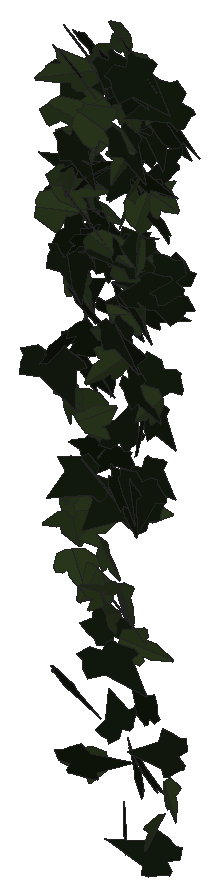
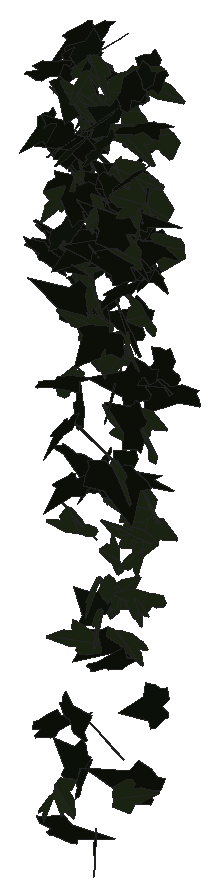
# SketchUp Ruby script. Lengths in inches.
U = 1.inch
M = Sketchup.active_model
def pt(a) = Geom::Point3d.new(a.map { |v| v * U })
def face(e, loops, mat)
  f = e.add_face(loops[0].map { |a| pt(a) })
  loops[1..].each { |l| e.add_face(l.map { |a| pt(a) }).erase! }
  f.material = f.back_material = mat if mat
  f
end
# faces: each face lists its corners as indices into pts; further lists are holes
def faces(e, pts, list, mat = nil) = list.each { |f| face(e, (f[0].is_a?(Array) ? f : [f]).map { |l| l.map { |i| pts[i] } }, mat) }
# xy, xz, yz: faces in a plane at the given z, y or x. An outline is a flat list of corners, or four numbers for a rectangle; further outlines are holes
def ring(l) = l.size == 4 ? [[l[0], l[1]], [l[2], l[1]], [l[2], l[3]], [l[0], l[3]]] : l.each_slice(2).to_a
def flat(e, list, mat, &to3) = list.each { |f| face(e, (f[0].is_a?(Array) ? f : [f]).map { |l| ring(l).map { |u, v| to3.(u, v) } }, mat) }
def xy(e, z, list, mat = nil) = flat(e, list, mat) { |x, y| [x, y, z] }
def xz(e, y, list, mat = nil) = flat(e, list, mat) { |x, z| [x, y, z] }
def yz(e, x, list, mat = nil) = flat(e, list, mat) { |y, z| [x, y, z] }
def lines(e, pts, list) = list.each { |a, b| e.add_line(pt(pts[a]), pt(pts[b])) }
# prism: a flat outline (further loops are holes) pulled along v
def prism(e, loops, v, mat = nil)
  f = face(e, loops, mat); d = Geom::Vector3d.new(v.map { |x| x * U })
  f.pushpull(f.normal.samedirection?(d) ? d.length : -d.length)
end
def box(e, o, s, mat = nil) = prism(e, [[o, [o[0] + s[0], o[1], o[2]], [o[0] + s[0], o[1] + s[1], o[2]], [o[0], o[1] + s[1], o[2]]]], [0, 0, s[2]], mat)
def at(x, y, z, deg = 0) = Geom::Transformation.translation(pt([x, y, z])) * Geom::Transformation.rotation(ORIGIN, Z_AXIS, deg.degrees)
def axes(o, x, y, z) = Geom::Transformation.new([*x, 0, *y, 0, *z, 0, *pt(o).to_a, 1])
def part(name) = M.definitions.add(name)
# library, detail: a bought-in or finely detailed component or shape, given as its bounding box
def library(name, o, s) = part(name).tap { |d| box(d.entities, o, s) }
def detail(e, o, s) = box(e.add_group.entities, o, s)
def put(e, d, t, mat = nil) = e.add_instance(d, t).tap { |i| i.material = mat if mat }
def group(e, t, mat = nil) = e.add_group.tap { |g| g.transformation = t; g.material = mat if mat }.entities
root = M.entities
M.materials.add("1026 AP 7946 SUNNY SIDE UP").color = [254, 231, 186]
M.materials.add("efeu1").color = [18, 25, 13]
M.materials.add("efeu2").color = [43, 57, 29]
c1 = part("ivyleaf_9")
p = [[1.54,2.16,1.25],[1.36,2.04,1.19],[-0.21,0.99,0.68],[-0.71,1.11,0.82],[-0.85,0.86,0.67],[-0.8,0.17,0.21],
  [-0.9,-0.01,0.1],[-0.67,-0.16,-0.02],[-0.08,-0.08,-0.05],[-0.03,-0.6,-0.4],[0.65,-0.88,-0.66],[0.83,-0.6,-0.49],
  [1.29,-0.42,-0.43],[1.8125,-0.07,-0.26],[1.21,0.44,0.15]]
faces(c1.entities,p,[[0,1,2,3,4,5,6,7,8,9,10,11,12,13,14]],"efeu1")
c2 = part("ivyleaf_10")
p = [[0,0.5,-0.03],[-0.0625,2.02,-0.43],[-0.19,2.01,-0.46],[-0.54,1.05,-0.29],[-0.52,0.625,-0.18],[-0.83,0.76,-0.28],
  [-1.16,0.64,-0.33],[-1.15,0.33,-0.24],[-0.77,-0.39,0.02],[-0.3,-0.51,0.16],[0.04,-0.48,0.23],[-0.02,2.01,-0.4375],
  [-0.06,2.01,-0.43],[0.04,-0.49,0.23],[0.67,-0.49,0.14],[1.38,0.36,-0.2],[1.375,0.51,-0.24],[0.81,0.65,-0.19],
  [0.62,0.59,-0.15],[0.6,1.09,-0.28],[0.5,1.23,-0.31]]
faces(c2.entities,p,[[0,1,2,3,4,5,6,7,8,9,10],[11,12,0,13,14,15,16,17,18,19,20]],"efeu2")
put(root,c1,axes([117.91,211.57,263.76],[-0.2339,-0.04974,-0.23344],[0.36038,0.008,-0.15696],[0.05363,-0.2707,0.03662]),"1026 AP 7946 SUNNY SIDE UP")
put(root,c2,axes([117.75,211.55,258.86],[0.19954,-0.17906,-0.13907],[0.1525,-0.09474,0.22452],[-0.31686,-0.15836,0.02048]),"1026 AP 7946 SUNNY SIDE UP")
put(root,c1,axes([119.03,211.49,266.57],[0.14137,-0.24472,-0.12578],[-0.08705,0.10808,-0.2676],[0.42014,0.10474,-0.01312]),"1026 AP 7946 SUNNY SIDE UP")
put(root,c1,axes([118.29,211.65,259.48],[-0.35679,-0.10894,0.10128],[-0.11872,-0.06989,-0.25808],[0.19862,-0.23747,0.02768]),"1026 AP 7946 SUNNY SIDE UP")
put(root,c2,axes([118.36,211.45,266.62],[0.19077,0.07882,0.31372],[0.46488,0.0815,-0.14281],[-0.16691,0.31708,-0.03919]),"1026 AP 7946 SUNNY SIDE UP")
put(root,c2,axes([118.03,211.64,267.4],[-0.1721,-0.05658,0.29739],[-0.33354,-0.19871,-0.124],[0.32119,-0.23667,0.03058]),"1026 AP 7946 SUNNY SIDE UP")
put(root,c1,axes([117.74,211.62,263.69],[0.0307,-0.27199,-0.04721],[-0.02149,0.04338,-0.28046],[0.43277,0.02145,-0.01058]),"1026 AP 7946 SUNNY SIDE UP")
put(root,c2,axes([117.94,211.52,258.58],[-0.33291,-0.20188,-0.04578],[0.07276,0.01403,-0.30048],[0.31639,-0.21565,0.02093]),"1026 AP 7946 SUNNY SIDE UP")
put(root,c1,axes([118.82,211.71,259.16],[-0.32164,-0.1641,0.08335],[-0.08027,-0.0668,-0.26982],[0.27695,-0.20994,0.0186]),"1026 AP 7946 SUNNY SIDE UP")
put(root,c2,axes([118.75,211.75,261.89],[-0.08754,-0.15593,0.27308],[-0.06137,-0.26453,-0.16974],[0.48088,-0.06214,0.02805]),"1026 AP 7946 SUNNY SIDE UP")
put(root,c1,axes([119.21,211.45,267.9375],[0.12735,-0.20008,-0.26303],[-0.07936,0.25101,-0.21864],[0.50241,0.09036,0.03214]),"1026 AP 7946 SUNNY SIDE UP")
put(root,c1,axes([117.72,211.51,267.65],[0.38751,-0.103,-0.07311],[-0.11037,0.01434,-0.27474],[0.16216,0.2559,-0.01229]),"1026 AP 7946 SUNNY SIDE UP")
put(root,c1,axes([117.83,211.6,266.02],[0.1422,-0.26206,-0.09408],[-0.06503,0.08067,-0.28484],[0.43071,0.09869,-0.01195]),"1026 AP 7946 SUNNY SIDE UP")
put(root,c1,axes([118.85,211.72,262.17],[0.01406,-0.04554,0.29639],[0.19039,-0.26149,-0.04801],[0.41701,0.12092,0.01193]),"1026 AP 7946 SUNNY SIDE UP")
put(root,c2,axes([119.3,211.66,262.95],[-0.28418,0.13219,0.17609],[0.21976,-0.09715,0.23008],[0.2579,0.22844,-0.00202]),"1026 AP 7946 SUNNY SIDE UP")
put(root,c2,axes([118.9,211.74,266.03],[-0.04369,-0.207,0.18217],[0.0845,-0.17957,-0.20753],[0.42088,0.01456,0.06058]),"1026 AP 7946 SUNNY SIDE UP")
put(root,c1,axes([117.87,211.42,264.32],[0.06788,-0.02547,-0.2658],[-0.16529,0.23722,-0.04088],[0.37241,0.10993,0.03031]),"1026 AP 7946 SUNNY SIDE UP")
put(root,c1,axes([117.36,211.62,261.54],[-0.16586,-0.19468,-0.20823],[0.17754,0.16696,-0.22664],[0.40262,-0.15383,0.01416]),"1026 AP 7946 SUNNY SIDE UP")
put(root,c1,axes([118.625,211.53,256.13],[-0.02783,-0.14577,-0.25507],[0.13322,0.23352,-0.14701],[0.43051,-0.08169,0.029]),"1026 AP 7946 SUNNY SIDE UP")
put(root,c1,axes([118.79,211.6,262.62],[0.12463,-0.235,-0.13116],[-0.08101,0.11545,-0.25458],[0.41136,0.09393,-0.0104]),"1026 AP 7946 SUNNY SIDE UP")
put(root,c1,axes([118.7,211.58,267.84],[0.19771,-0.22892,-0.13375],[-0.01614,0.13812,-0.26296],[0.4125,0.11513,0.05382]),"1026 AP 7946 SUNNY SIDE UP")
put(root,c1,axes([118.2,211.61,259.62],[0.39579,-0.15458,-0.02055],[-0.04465,-0.00991,-0.30342],[0.24081,0.25224,-0.02249]),"1026 AP 7946 SUNNY SIDE UP")
put(root,c1,axes([117.77,211.63,264.85],[0.39505,-0.19066,-0.0237],[-0.04918,-0.00504,-0.32409],[0.29774,0.25214,-0.02208]),"1026 AP 7946 SUNNY SIDE UP")
put(root,c2,axes([118.55,211.7,256.8],[-0.21713,0.08438,0.21135],[0.28906,-0.09071,0.16577],[0.19397,0.22963,-0.01045]),"1026 AP 7946 SUNNY SIDE UP")
put(root,c1,axes([118.93,211.75,263.19],[0.17493,-0.23959,0.08885],[0.05647,-0.07991,-0.2726],[0.39714,0.1169,-0.00037]),"1026 AP 7946 SUNNY SIDE UP")
put(root,c1,axes([119.88,211.75,263.62],[-0.00599,-0.04521,-0.31222],[-0.27328,-0.24899,0.03909],[-0.39633,0.17237,-0.02224]),"1026 AP 7946 SUNNY SIDE UP")
put(root,c2,axes([118.42,211.63,264.18],[-0.23635,-0.02607,-0.22702],[0.34709,-0.04309,-0.15021],[-0.03343,-0.26313,0.0455]),"1026 AP 7946 SUNNY SIDE UP")
put(root,c1,axes([117.51,211.4,261.74],[0.09602,0.1278,0.24119],[0.18233,0.20275,-0.14444],[-0.3766,0.13075,-0.00843]),"1026 AP 7946 SUNNY SIDE UP")
put(root,c2,axes([118.47,211.8,257.11],[-0.13149,-0.09902,-0.23315],[-0.20997,-0.1822,0.13222],[-0.32583,0.15737,0.00889]),"1026 AP 7946 SUNNY SIDE UP")
put(root,c1,axes([117.51,211.68,255.22],[0.34123,-0.13918,0.06616],[0.06798,-0.05265,-0.26507],[0.23178,0.22034,-0.01967]),"1026 AP 7946 SUNNY SIDE UP")
put(root,c1,axes([118.86,211.77,259.36],[-0.13825,-0.04099,-0.26517],[0.40926,-0.02253,-0.0881],[-0.01312,-0.27084,0.04583]),"1026 AP 7946 SUNNY SIDE UP")
put(root,c1,axes([119.25,211.77,259.6],[-0.32098,-0.08866,-0.16968],[0.25905,0.02868,-0.22678],[0.13781,-0.2604,0.03107]),"1026 AP 7946 SUNNY SIDE UP")
put(root,c2,axes([119.23,211.81,264.31],[0.00296,0.17756,-0.22157],[0.01397,-0.21601,-0.18405],[-0.43954,-0.00567,-0.00734]),"1026 AP 7946 SUNNY SIDE UP")
put(root,c1,axes([119.1,211.57,265.68],[-0.27333,0.22878,0.12627],[-0.13575,0.0865,-0.29509],[-0.38386,-0.1935,0.01444]),"1026 AP 7946 SUNNY SIDE UP")
put(root,c2,axes([117.85,211.74,265.35],[-0.02198,-0.28236,0.03978],[-0.00139,-0.04022,-0.29147],[0.44846,-0.01396,0.00105]),"1026 AP 7946 SUNNY SIDE UP")
put(root,c1,axes([118.77,211.62,259.57],[0.27263,-0.15613,-0.19249],[-0.21315,0.12734,-0.2396],[0.31676,0.22007,0.00444]),"1026 AP 7946 SUNNY SIDE UP")
put(root,c1,axes([117.84,211.81,262.6875],[0.24059,-0.16282,0.16392],[0.15579,-0.12621,-0.23061],[0.32342,0.18192,-0.01085]),"1026 AP 7946 SUNNY SIDE UP")
put(root,c2,axes([117.59,211.65,264.95],[-0.16145,-0.02403,0.29429],[0.40773,0.12193,0.10725],[-0.19269,0.27813,-0.01964]),"1026 AP 7946 SUNNY SIDE UP")
put(root,c2,axes([118.35,211.82,257.92],[0.09327,-0.05987,0.25327],[0.35427,-0.1032,-0.08238],[0.18224,0.23125,0.03052]),"1026 AP 7946 SUNNY SIDE UP")
put(root,c2,axes([117.48,211.65,266.49],[-0.21945,-0.07434,-0.23151],[0.34202,0.06137,-0.16002],[0.14517,-0.25695,0.02704]),"1026 AP 7946 SUNNY SIDE UP")
put(root,c1,axes([119.08,211.68,261.61],[0.22561,-0.1844,-0.15661],[-0.12548,0.12888,-0.23954],[0.3531,0.16361,0.01494]),"1026 AP 7946 SUNNY SIDE UP")
put(root,c1,axes([119.15,211.84,260.39],[0.01862,0.12503,0.25884],[-0.09542,-0.24366,0.1268],[0.42983,-0.05951,0.01694]),"1026 AP 7946 SUNNY SIDE UP")
put(root,c2,axes([118.91,211.75,263.73],[-0.06854,-0.03092,-0.31335],[0.47264,-0.05954,-0.03851],[-0.08637,-0.30127,0.03792]),"1026 AP 7946 SUNNY SIDE UP")
put(root,c2,axes([117.99,211.5625,258.93],[-0.04722,-0.12702,0.28388],[0.10947,0.26738,0.136],[-0.46544,0.07577,0.00318]),"1026 AP 7946 SUNNY SIDE UP")
put(root,c2,axes([119.3125,211.55,264.94],[0.08346,0.15417,-0.2369],[0.04793,0.23036,0.16707],[0.43383,-0.05511,0.02712]),"1026 AP 7946 SUNNY SIDE UP")
put(root,c1,axes([119.25,211.81,264.08],[-0.34642,0.05611,0.17098],[-0.26791,-0.00872,-0.23045],[-0.06207,-0.2755,0.04044]),"1026 AP 7946 SUNNY SIDE UP")
put(root,c2,axes([117.93,211.68,258.36],[0.21302,-0.03813,-0.23827],[0.36354,0.06434,0.12908],[0.05872,-0.26002,0.06524]),"1026 AP 7946 SUNNY SIDE UP")
put(root,c1,axes([119.23,211.62,267.49],[0.02909,-0.08916,-0.27424],[-0.14315,0.24993,-0.09147],[0.41678,0.09206,-0.01228]),"1026 AP 7946 SUNNY SIDE UP")
put(root,c1,axes([118.69,211.94,256.77],[0.09933,-0.16924,0.21382],[0.13425,-0.19043,-0.18699],[0.40036,0.10585,0.00965]),"1026 AP 7946 SUNNY SIDE UP")
put(root,c1,axes([118.52,211.72,264.32],[0.04961,-0.01399,-0.30866],[-0.46773,-0.03948,-0.03061],[-0.05952,0.2986,-0.01673]),"1026 AP 7946 SUNNY SIDE UP")
put(root,c1,axes([118.19,211.73,265.54],[0.14498,0.22879,-0.14867],[-0.07125,-0.13863,-0.25478],[-0.42044,0.10239,-0.00809]),"1026 AP 7946 SUNNY SIDE UP")
put(root,c2,axes([118.01,211.8,260.44],[0.29325,-0.0875,-0.19247],[0.29011,-0.04047,0.20958],[-0.14357,-0.26051,0.03036]),"1026 AP 7946 SUNNY SIDE UP")
put(root,c1,axes([119.92,211.8,263.84],[-0.39878,0.12931,0.11719],[-0.18004,0.02292,-0.29157],[-0.20127,-0.27671,0.02863]),"1026 AP 7946 SUNNY SIDE UP")
put(root,c1,axes([117.97,211.61,263.9375],[0.23996,0.12091,0.20328],[0.26879,0.09922,-0.19894],[-0.24393,0.22828,-0.01924]),"1026 AP 7946 SUNNY SIDE UP")
put(root,c1,axes([118.98,211.875,265.64],[0.20414,-0.08209,0.2155],[0.23792,-0.14739,-0.15685],[0.26216,0.19769,-0.02546]),"1026 AP 7946 SUNNY SIDE UP")
put(root,c2,axes([119.36,212.02,261.13],[-0.08777,-0.02999,0.27951],[0.09868,-0.27109,-0.01914],[0.41799,0.0577,0.06321]),"1026 AP 7946 SUNNY SIDE UP")
put(root,c2,axes([117.91,211.8125,260.89],[-0.39344,-0.09878,0.00288],[0.00915,-0.02386,-0.27614],[0.15514,-0.2491,0.02361]),"1026 AP 7946 SUNNY SIDE UP")
put(root,c2,axes([119.5,211.93,252.93],[0.06406,-0.25149,0.11289],[0.03689,-0.10863,-0.26304],[0.43067,0.04671,0.00574]),"1026 AP 7946 SUNNY SIDE UP")
put(root,c2,axes([117.22,211.73,264.39],[0.00587,-0.05817,-0.31077],[0.44323,0.11982,-0.01953],[0.19084,-0.27651,0.05492]),"1026 AP 7946 SUNNY SIDE UP")
put(root,c1,axes([117.74,211.78,253.52],[0.12261,0.009,0.26705],[0.40775,0.00005,-0.08038],[-0.00415,0.27065,-0.00728]),"1026 AP 7946 SUNNY SIDE UP")
put(root,c1,axes([118.04,211.78,265.09],[0.1597,0.2799,0.01791],[-0.03473,-0.00876,0.30615],[0.43945,-0.10241,0.01769]),"1026 AP 7946 SUNNY SIDE UP")
put(root,c2,axes([117.63,211.97,263.01],[0.2568,-0.04491,0.21797],[0.31689,-0.06554,-0.17477],[0.12457,0.25933,-0.00476]),"1026 AP 7946 SUNNY SIDE UP")
put(root,c2,axes([118.01,211.94,257.3],[0.37437,-0.12969,-0.00363],[-0.02113,-0.01886,-0.27841],[0.20288,0.23735,-0.02229]),"1026 AP 7946 SUNNY SIDE UP")
put(root,c1,axes([119.8,212.1,267.1875],[-0.30841,-0.11677,0.17947],[-0.21857,-0.10743,-0.23515],[0.24809,-0.23981,0.01594]),"1026 AP 7946 SUNNY SIDE UP")
put(root,c1,axes([119.62,211.95,252.18],[-0.19094,0.04528,0.23866],[-0.36454,0.02459,-0.13014],[-0.06768,-0.26017,0.02765]),"1026 AP 7946 SUNNY SIDE UP")
put(root,c2,axes([117.39,212.07,260.5],[0.01401,-0.07695,-0.26325],[0.19118,-0.22594,0.07326],[-0.3728,-0.11876,0.02768]),"1026 AP 7946 SUNNY SIDE UP")
put(root,c1,axes([118.83,212.0625,267.46],[-0.19475,-0.02322,-0.251],[0.37452,-0.07364,-0.118],[-0.08765,-0.26309,0.05351]),"1026 AP 7946 SUNNY SIDE UP")
put(root,c2,axes([118.82,211.85,257.18],[-0.13908,0.25231,0.05638],[-0.0463,0.0461,-0.27488],[-0.40283,-0.09241,0.01213]),"1026 AP 7946 SUNNY SIDE UP")
put(root,c2,axes([118.83,211.92,266.83],[-0.26135,-0.20894,-0.06411],[0.0859,0.03431,-0.27401],[0.33132,-0.17371,0.02047]),"1026 AP 7946 SUNNY SIDE UP")
put(root,c1,axes([119.73,212.13,254.2],[-0.13261,-0.04453,0.25458],[-0.3017,-0.15713,-0.09745],[0.25528,-0.20884,0.01707]),"1026 AP 7946 SUNNY SIDE UP")
put(root,c1,axes([118.98,212.12,253.71],[0.0996,-0.12773,0.22505],[0.13537,-0.20168,-0.14789],[0.37522,0.10666,-0.00638]),"1026 AP 7946 SUNNY SIDE UP")
put(root,c2,axes([117.61,211.96,257.47],[0.30301,0.17699,0.06129],[0.08491,0.0275,-0.26889],[-0.28053,0.1995,-0.01519]),"1026 AP 7946 SUNNY SIDE UP")
put(root,c2,axes([117.98,212.15,253.47],[0.0141,-0.02234,-0.26486],[-0.29325,-0.17818,0.00821],[-0.28018,0.18538,-0.02193]),"1026 AP 7946 SUNNY SIDE UP")
put(root,c1,axes([118.68,212.14,267.85],[0.19377,-0.20634,0.14938],[0.08681,-0.13673,-0.24759],[0.38803,0.13363,-0.01921]),"1026 AP 7946 SUNNY SIDE UP")
put(root,c1,axes([118.33,211.93,263.45],[-0.1844,0.20267,0.11785],[0.08816,-0.09839,0.24065],[0.35425,0.12998,0.00145]),"1026 AP 7946 SUNNY SIDE UP")
put(root,c1,axes([117.52,212.125,267.62],[0.24523,-0.20428,0.12533],[0.09223,-0.10937,-0.26477],[0.36327,0.16567,-0.01738]),"1026 AP 7946 SUNNY SIDE UP")
put(root,c2,axes([117.69,212.16,264.89],[-0.1237,0.09419,-0.24984],[0.1562,-0.22389,-0.12381],[-0.37894,-0.12303,0.03052]),"1026 AP 7946 SUNNY SIDE UP")
put(root,c1,axes([118.125,211.88,263.98],[0.19337,0.03848,0.26756],[0.38925,0.07783,-0.13229],[-0.13652,0.27642,0.00179]),"1026 AP 7946 SUNNY SIDE UP")
put(root,c2,axes([119,211.82,265.18],[0.08406,-0.06862,0.31256],[-0.1628,0.28678,0.08719],[-0.46186,-0.11357,0.02615]),"1026 AP 7946 SUNNY SIDE UP")
put(root,c1,axes([117.49,212.15,264.59],[-0.31302,-0.13451,-0.12656],[0.1751,0.05274,-0.24661],[0.22567,-0.22749,0.01579]),"1026 AP 7946 SUNNY SIDE UP")
put(root,c2,axes([117.97,212.08,266.59],[0.3784,-0.06987,-0.16186],[-0.24318,0.02861,-0.25762],[0.11687,0.28575,-0.012]),"1026 AP 7946 SUNNY SIDE UP")
put(root,c2,axes([118.06,212.27,267.45],[0.03016,0.04947,-0.28228],[-0.21414,-0.23822,-0.05547],[-0.38237,0.13731,0.0088]),"1026 AP 7946 SUNNY SIDE UP")
put(root,c2,axes([118.8125,212.01,256.18],[0.0541,0.0418,0.27184],[0.36778,0.12336,-0.05087],[-0.20224,0.23552,-0.0198]),"1026 AP 7946 SUNNY SIDE UP")
put(root,c2,axes([117.9375,212.21,265.81],[0.23026,-0.1859,0.13865],[0.10744,-0.11841,-0.24386],[0.34554,0.1607,-0.01658]),"1026 AP 7946 SUNNY SIDE UP")
put(root,c2,axes([118.67,212.24,264.86],[0.11848,-0.20776,0.16028],[0.08333,-0.14753,-0.22854],[0.40067,0.09212,0.00013]),"1026 AP 7946 SUNNY SIDE UP")
put(root,c1,axes([118.78,211.9,264.07],[0.01102,-0.00142,-0.30152],[-0.08233,0.28803,-0.00105],[0.45279,0.05241,0.00715]),"1026 AP 7946 SUNNY SIDE UP")
put(root,c1,axes([118.43,212.05,265.36],[0.30642,0.04094,-0.19711],[-0.27917,-0.07725,-0.20353],[-0.13014,0.26212,-0.02749]),"1026 AP 7946 SUNNY SIDE UP")
put(root,c1,axes([118.84,212.13,262.79],[0.13492,-0.02664,0.26938],[0.35634,-0.13215,-0.0912],[0.20983,0.24156,-0.01833]),"1026 AP 7946 SUNNY SIDE UP")
put(root,c1,axes([118.99,212.3125,266.08],[-0.01346,-0.02871,-0.2793],[0.11767,-0.26091,0.02452],[-0.41195,-0.07358,0.01613]),"1026 AP 7946 SUNNY SIDE UP")
put(root,c2,axes([118.68,212.01,267.55],[-0.18047,-0.25592,-0.20323],[0.19519,0.15671,-0.28503],[0.46758,-0.16419,0.04055]),"1026 AP 7946 SUNNY SIDE UP")
put(root,c1,axes([118.15,212.09,259.79],[0.26025,0.13447,-0.21263],[-0.23348,-0.1451,-0.22009],[-0.31034,0.22194,-0.01273]),"1026 AP 7946 SUNNY SIDE UP")
put(root,c1,axes([117.54,212.3,266.93],[-0.2653,-0.21169,0.03169],[-0.00783,-0.0368,-0.27841],[0.33654,-0.16774,0.0185]),"1026 AP 7946 SUNNY SIDE UP")
put(root,c1,axes([118.625,211.98,254.45],[-0.32513,0.08506,-0.15233],[-0.2089,0.06666,0.23053],[0.1693,0.2456,-0.0081]),"1026 AP 7946 SUNNY SIDE UP")
put(root,c1,axes([118.1,212.37,261.17],[-0.01799,-0.02333,0.31368],[-0.10852,-0.29676,-0.02782],[0.46798,-0.06971,0.00561]),"1026 AP 7946 SUNNY SIDE UP")
put(root,c1,axes([119.66,212.15,265.93],[-0.30522,0.17594,-0.04167],[0.02809,-0.04185,-0.26944],[-0.28283,-0.19403,0.01821]),"1026 AP 7946 SUNNY SIDE UP")
put(root,c1,axes([117.65,212.22,262.54],[-0.03142,0.14515,0.23876],[0.0614,-0.22765,0.14956],[0.42449,0.04367,-0.00396]),"1026 AP 7946 SUNNY SIDE UP")
put(root,c2,axes([117.91,212.2,265.9],[0.14596,-0.00682,-0.24702],[-0.37664,-0.01569,-0.09517],[-0.01915,0.25661,-0.01088]),"1026 AP 7946 SUNNY SIDE UP")
put(root,c1,axes([117.7,212.29,267.44],[0.08343,-0.11465,0.24681],[0.22627,-0.19372,-0.12912],[0.35212,0.15165,0.02449]),"1026 AP 7946 SUNNY SIDE UP")
put(root,c1,axes([118.58,212.01,260.11],[-0.32522,0.20422,0.02403],[0.04186,-0.00454,0.29899],[0.32028,0.20796,-0.01468]),"1026 AP 7946 SUNNY SIDE UP")
put(root,c2,axes([118.68,212.18,266.89],[0.06834,-0.0862,-0.24738],[0.39168,-0.03621,0.05975],[-0.08336,-0.24085,0.07794]),"1026 AP 7946 SUNNY SIDE UP")
put(root,c1,axes([118.95,212.125,253.35],[0.00996,-0.17441,0.20023],[0.03447,0.19507,0.17983],[-0.41033,0.01216,0.01997]),"1026 AP 7946 SUNNY SIDE UP")
put(root,c2,axes([118.1,212.38,261.96],[-0.03089,-0.10743,-0.25966],[-0.11197,-0.24138,0.11056],[-0.4151,0.0731,-0.0105]),"1026 AP 7946 SUNNY SIDE UP")
put(root,c1,axes([117.87,212.21,265.04],[-0.18114,0.05515,0.23126],[-0.34542,0.05081,-0.12888],[-0.11157,-0.24686,0.02356]),"1026 AP 7946 SUNNY SIDE UP")
put(root,c1,axes([119.75,212.14,263.57],[-0.17433,0.10641,0.23897],[-0.30313,0.1298,-0.15591],[-0.26163,-0.22129,0.02142]),"1026 AP 7946 SUNNY SIDE UP")
put(root,c2,axes([118.47,212.15,262.54],[0.16464,-0.02127,-0.2612],[0.39655,0.04407,0.10379],[0.05163,-0.27064,0.03579]),"1026 AP 7946 SUNNY SIDE UP")
put(root,c1,axes([117.59,212.05,261.69],[0.08262,0.0678,0.28232],[0.38621,0.12566,-0.07992],[-0.21765,0.24872,-0.03465]),"1026 AP 7946 SUNNY SIDE UP")
put(root,c1,axes([117.73,212.3,264.11],[0.28729,-0.09618,0.17992],[0.21241,-0.11551,-0.21113],[0.2316,0.22524,-0.02954]),"1026 AP 7946 SUNNY SIDE UP")
put(root,c2,axes([117.57,212.3,265.24],[-0.21168,0.17437,-0.14178],[0.11756,-0.11719,-0.22737],[-0.32994,-0.15363,0.00995]),"1026 AP 7946 SUNNY SIDE UP")
put(root,c2,axes([117.63,212.37,262.54],[0.22225,-0.1799,0.13236],[0.12715,-0.10116,-0.23628],[0.32452,0.16284,0.00193]),"1026 AP 7946 SUNNY SIDE UP")
put(root,c2,axes([117.625,212.29,264.35],[0.00567,0.01017,0.27698],[0.42272,0.00924,-0.00402],[-0.01475,0.26867,-0.00877]),"1026 AP 7946 SUNNY SIDE UP")
put(root,c1,axes([118.07,212.29,265.73],[-0.19403,0.21367,-0.12391],[0.07523,-0.11246,-0.25448],[-0.3791,-0.13168,0.01291]),"1026 AP 7946 SUNNY SIDE UP")
put(root,c1,axes([119.11,212.12,258.6875],[-0.3225,0.08488,-0.15764],[-0.20924,0.07856,0.22839],[0.17969,0.24383,-0.01697]),"1026 AP 7946 SUNNY SIDE UP")
put(root,c1,axes([118.25,212.21,262.58],[0.42565,0.03435,-0.04388],[-0.06124,-0.03143,-0.28002],[-0.06077,0.27225,-0.02515]),"1026 AP 7946 SUNNY SIDE UP")
put(root,c2,axes([119.18,212.19,266.97],[0.10782,-0.08834,-0.28868],[-0.34858,0.17252,-0.1111],[0.30206,0.23062,-0.02517]),"1026 AP 7946 SUNNY SIDE UP")
put(root,c2,axes([118.44,212.2,256.87],[-0.18782,0.20816,0.10035],[-0.10553,0.07202,-0.2459],[-0.34481,-0.13543,0.02059]),"1026 AP 7946 SUNNY SIDE UP")
put(root,c1,axes([118.32,212.46,252.42],[-0.01191,-0.02343,-0.26889],[0.35784,-0.12979,0.00444],[-0.20389,-0.22643,0.0235]),"1026 AP 7946 SUNNY SIDE UP")
put(root,c1,axes([117.38,212.4375,261.09],[0.19959,-0.04191,-0.27968],[0.42635,-0.02719,0.13489],[-0.06692,-0.29824,0.02521]),"1026 AP 7946 SUNNY SIDE UP")
put(root,c1,axes([117.61,212.52,265.93],[-0.11369,-0.1963,0.15852],[-0.07081,-0.14848,-0.21625],[0.38685,-0.08487,0.007]),"1026 AP 7946 SUNNY SIDE UP")
put(root,c1,axes([118.2,212.29,256.03],[-0.29458,-0.14632,0.10788],[0.10951,0.08172,0.24452],[-0.26169,0.1989,-0.01911]),"1026 AP 7946 SUNNY SIDE UP")
put(root,c1,axes([118.83,212.29,265.29],[0.32727,0.10427,-0.14587],[-0.17537,-0.09253,-0.23862],[-0.21474,0.23447,-0.02744]),"1026 AP 7946 SUNNY SIDE UP")
put(root,c2,axes([118.01,212.25,259.9375],[0.14531,-0.15328,-0.21644],[-0.18026,0.1751,-0.18329],[0.36582,0.14716,-0.00434]),"1026 AP 7946 SUNNY SIDE UP")
put(root,c1,axes([119.125,212.52,261.46],[-0.24555,-0.20758,0.04069],[-0.01552,-0.04335,-0.26722],[0.33224,-0.15544,0.01759]),"1026 AP 7946 SUNNY SIDE UP")
put(root,c1,axes([119.1,212.15,266.93],[0.06481,0.1837,0.1877],[-0.00783,0.18398,-0.18995],[-0.40559,0.0258,0.03366]),"1026 AP 7946 SUNNY SIDE UP")
put(root,c1,axes([117.76,212.3125,263.71],[0.13231,-0.17432,-0.18845],[-0.05647,0.18155,-0.19526],[0.39215,0.08496,0.03546]),"1026 AP 7946 SUNNY SIDE UP")
put(root,c1,axes([118.9,212.52,266.23],[0.03828,-0.25187,0.0448],[0.01423,-0.04424,-0.2609],[0.40204,0.02555,0.00497]),"1026 AP 7946 SUNNY SIDE UP")
put(root,c1,axes([118.98,212.28,254.69],[0.03582,-0.02709,0.26754],[-0.14192,0.24396,0.03578],[-0.38552,-0.09233,0.01169]),"1026 AP 7946 SUNNY SIDE UP")
put(root,c2,axes([117.5625,212.21,258.45],[0.00904,-0.03401,-0.26984],[0.08761,0.25606,-0.03152],[0.40567,-0.05454,0.01282]),"1026 AP 7946 SUNNY SIDE UP")
put(root,c2,axes([117.72,212.45,256.86],[0.37312,-0.06387,-0.07991],[-0.1258,-0.00128,-0.25224],[0.09486,0.24953,-0.02019]),"1026 AP 7946 SUNNY SIDE UP")
put(root,c1,axes([117.93,212.57,266.99],[0.14826,-0.1898,0.17535],[0.12057,-0.15317,-0.21922],[0.3835,0.12153,0.00113]),"1026 AP 7946 SUNNY SIDE UP")
put(root,c2,axes([118.4,212.35,267.9],[0.25956,-0.14101,-0.17285],[-0.148,0.14299,-0.21942],[0.31015,0.18624,0.03996]),"1026 AP 7946 SUNNY SIDE UP")
put(root,c1,axes([118.85,212.64,264.4375],[0.27353,-0.23018,-0.11861],[0.13181,-0.07905,0.29619],[-0.38165,-0.19227,0.01729]),"1026 AP 7946 SUNNY SIDE UP")
put(root,c1,axes([118.85,212.35,259.5],[0.0566,-0.12305,-0.23421],[-0.08598,0.22,-0.13071],[0.3963,0.0653,0.00509]),"1026 AP 7946 SUNNY SIDE UP")
put(root,c1,axes([118.04,212.67,267.03],[-0.0818,-0.20393,0.16773],[-0.01395,-0.16571,-0.21619],[0.41122,-0.04619,0.02603]),"1026 AP 7946 SUNNY SIDE UP")
put(root,c1,axes([118.06,212.61,266.45],[0.13346,-0.24303,0.07036],[0.02702,-0.06779,-0.26553],[0.39663,0.0864,-0.00559]),"1026 AP 7946 SUNNY SIDE UP")
put(root,c1,axes([118.99,212.41,260.61],[0.12964,-0.16442,-0.19276],[-0.15468,0.15851,-0.18816],[0.35863,0.1278,-0.01148]),"1026 AP 7946 SUNNY SIDE UP")
put(root,c2,axes([118.75,212.42,258.61],[0.39592,0.05724,-0.04405],[0.05084,0.0497,0.26297],[0.10052,-0.25057,0.0405]),"1026 AP 7946 SUNNY SIDE UP")
put(root,c2,axes([119.13,212.32,265.01],[0.03056,0.18627,0.20783],[0.00025,0.20118,-0.19121],[-0.43054,0.01334,0.01464]),"1026 AP 7946 SUNNY SIDE UP")
put(root,c1,axes([118.81,212.48,266.43],[-0.06153,-0.04854,-0.28193],[0.34162,0.16658,-0.06153],[0.27188,-0.22029,0.01351]),"1026 AP 7946 SUNNY SIDE UP")
put(root,c2,axes([118.51,212.35,263.39],[-0.05755,0.04672,0.28966],[-0.36458,0.15952,-0.05752],[-0.25994,-0.23409,0.01656]),"1026 AP 7946 SUNNY SIDE UP")
put(root,c2,axes([117.54,212.33,265.46],[0.01175,-0.15645,0.25743],[-0.02656,0.25021,0.1628],[-0.464,-0.01829,-0.0028]),"1026 AP 7946 SUNNY SIDE UP")
put(root,c2,axes([118.25,212.31,265],[0.08945,0.01355,0.27167],[-0.11866,0.25927,0.00456],[-0.39777,-0.0743,0.05973]),"1026 AP 7946 SUNNY SIDE UP")
put(root,c1,axes([118.65,212.66,266.25],[0.08804,-0.24795,0.07762],[0.01229,-0.07687,-0.26215],[0.40794,0.05583,-0.00885]),"1026 AP 7946 SUNNY SIDE UP")
put(root,c1,axes([117.61,212.55,264.91],[0.3123,0.03373,-0.1601],[0.21983,0.08208,0.20265],[0.11979,-0.23858,0.0455]),"1026 AP 7946 SUNNY SIDE UP")
put(root,c2,axes([119.24,212.52,253.19],[-0.07808,0.26128,-0.00173],[-0.00644,-0.004,-0.27396],[-0.41081,-0.0496,0.00462]),"1026 AP 7946 SUNNY SIDE UP")
put(root,c1,axes([119.27,212.52,266.49],[0.30948,-0.13589,-0.10258],[-0.12063,0.0627,-0.24591],[0.23504,0.21111,0.00886]),"1026 AP 7946 SUNNY SIDE UP")
